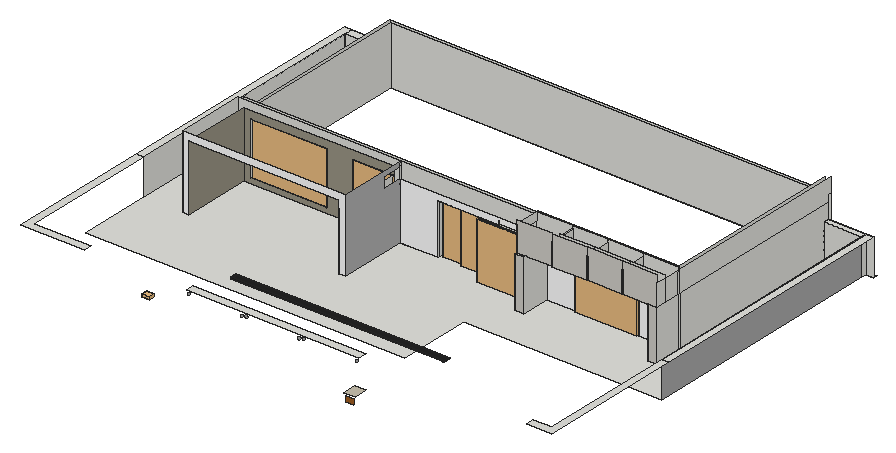
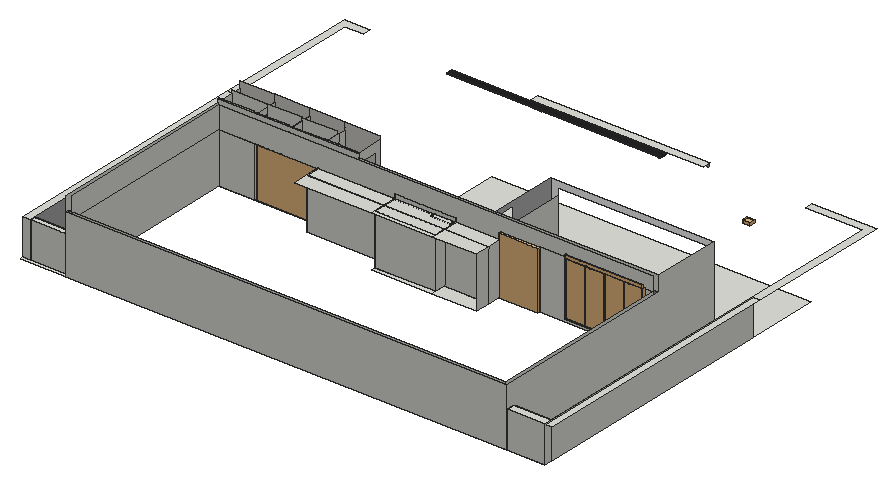
# SketchUp Ruby script. Lengths in inches.
U = 1.inch
M = Sketchup.active_model
def pt(a) = Geom::Point3d.new(a.map { |v| v * U })
def face(e, loops, mat)
  f = e.add_face(loops[0].map { |a| pt(a) })
  loops[1..].each { |l| e.add_face(l.map { |a| pt(a) }).erase! }
  f.material = f.back_material = mat if mat
  f
end
# faces: each face lists its corners as indices into pts; further lists are holes
def faces(e, pts, list, mat = nil) = list.each { |f| face(e, (f[0].is_a?(Array) ? f : [f]).map { |l| l.map { |i| pts[i] } }, mat) }
# xy, xz, yz: faces in a plane at the given z, y or x. An outline is a flat list of corners, or four numbers for a rectangle; further outlines are holes
def ring(l) = l.size == 4 ? [[l[0], l[1]], [l[2], l[1]], [l[2], l[3]], [l[0], l[3]]] : l.each_slice(2).to_a
def flat(e, list, mat, &to3) = list.each { |f| face(e, (f[0].is_a?(Array) ? f : [f]).map { |l| ring(l).map { |u, v| to3.(u, v) } }, mat) }
def xy(e, z, list, mat = nil) = flat(e, list, mat) { |x, y| [x, y, z] }
def xz(e, y, list, mat = nil) = flat(e, list, mat) { |x, z| [x, y, z] }
def yz(e, x, list, mat = nil) = flat(e, list, mat) { |y, z| [x, y, z] }
def lines(e, pts, list) = list.each { |a, b| e.add_line(pt(pts[a]), pt(pts[b])) }
# prism: a flat outline (further loops are holes) pulled along v
def prism(e, loops, v, mat = nil)
  f = face(e, loops, mat); d = Geom::Vector3d.new(v.map { |x| x * U })
  f.pushpull(f.normal.samedirection?(d) ? d.length : -d.length)
end
def box(e, o, s, mat = nil) = prism(e, [[o, [o[0] + s[0], o[1], o[2]], [o[0] + s[0], o[1] + s[1], o[2]], [o[0], o[1] + s[1], o[2]]]], [0, 0, s[2]], mat)
def at(x, y, z, deg = 0) = Geom::Transformation.translation(pt([x, y, z])) * Geom::Transformation.rotation(ORIGIN, Z_AXIS, deg.degrees)
def axes(o, x, y, z) = Geom::Transformation.new([*x, 0, *y, 0, *z, 0, *pt(o).to_a, 1])
def part(name) = M.definitions.add(name)
# library, detail: a bought-in or finely detailed component or shape, given as its bounding box
def library(name, o, s) = part(name).tap { |d| box(d.entities, o, s) }
def detail(e, o, s) = box(e.add_group.entities, o, s)
def put(e, d, t, mat = nil) = e.add_instance(d, t).tap { |i| i.material = mat if mat }
def group(e, t, mat = nil) = e.add_group.tap { |g| g.transformation = t; g.material = mat if mat }.entities
root = M.entities
M.materials.add("Material~3").color = [123, 113, 102]
M.materials.add("[0128_White]").color = [255, 255, 255]
M.materials.add("[0129_WhiteSmoke]").color = [178, 178, 178]
M.materials.add("[0132_LightGray]").color = [169, 169, 169]
M.materials.add("[0136_Charcoal]").color = [35, 35, 35]
M.materials.add("[Concrete Tile]").color = [155, 150, 134]
M.materials.add("[Terrazzo Tile Light]").color = [209, 207, 200]
M.materials.add("[Tile Canvas]").color = [199, 192, 173]
M.materials.add("[Wood Square Tile 02]").color = [160, 95, 34]
M.materials.add("terracota").color = [125, 74, 68]
c1 = library("3DGeom~4_Defintion",[362.52,-15.59,12.6],[288.85,70.11,1000])
c2 = library("3 door",[0,0,0],[74.8,3.9375,43.31])
c3 = library("Shallow planter bowl",[0,0,0],[21.33,16.65,7.48])
c4 = library("door (1)",[38.93,25.48,0],[40,9.94,82.68])
c5 = part("Group\#105")
prism(c5.entities,[[[353.71,0,0.79],[353.71,0,-1.18],[353.71,10.43,-1.18],[353.71,10.43,0.79],[353.71,10.12,0.79],[353.71,10.12,0.39],[353.71,7.09,0.39],[353.71,7.09,0.79],[353.71,6.73,0.79],[353.71,6.73,0.39],[353.71,3.7,0.39],[353.71,3.7,0.79],[353.71,3.35,0.79],[353.71,3.35,0.39],[353.71,0.31,0.39],[353.71,0.31,0.79]]],[-353.71,0,0])
c6 = library("JALI+PATTERN-03",[8.875,53.125,6.4375],[84,1,53.5])
xy(root,5.1875,[[[2928.38,611.53,3456.29,611.53,3456.29,732.28,3784.01,732.28,3784.01,1146.63,3720.76,1146.63,3720.76,851.0625,3551.34,851.0625,3551.34,845.35,3503.88,845.35,3503.88,798.41,3488.55,798.41,3488.55,845.35,3424.27,845.35,3424.27,874.25,3323.99,874.25,3323.99,845.35,3261.3,845.35,3261.3,732.28,3250.36,732.28,3250.36,851.0625,3184.99,851.0625,3184.99,845.35,3002.95,845.35,3002.95,732.28,2992.01,732.28,2992.01,1146.63,2928.38,1146.63],[3705.43,801.78,3720.76,845.35]],[2992.01,732.28,2992.01,1160.85,3796.01,1160.85,3796.01,1155.13,2997.72,1155.13,2997.72,851.0625,3184.99,851.0625,3184.99,845.35,3002.95,845.35,3002.95,732.28],[3250.36,732.28,3250.36,846.1,3323.99,846.1,3323.99,845.35,3261.3,845.35,3261.3,732.28],[3488.55,798.41,3488.55,845.35,3424.27,845.35,3424.27,846.1,3551.34,846.1,3551.34,845.35,3503.88,845.35,3503.88,798.41],[3705.43,801.78,3720.76,845.35],
  [3250.36,846.1,3323.99,874.25],[3424.27,846.1,3551.34,874.25],[3715.04,851.0625,3720.76,1155.13],[3250.36,874.25,3323.99,900.375],[3323.99,874.25,3424.27,892.35],
  [3323.99,892.35,3424.27,900.375],[2928.38,1146.63,2992.01,1160.85],[3720.76,1146.63,3784.01,1155.13]])
xy(root,13.84,[[3014.67,845.35,3139.54,851.0625]])
xy(root,32.74,[[3482.52,453.42,3500.96,475.99]],"[Tile Canvas]")
xy(root,65.1875,[[2916.76,491.47,3022.65,491.47,3022.65,505.1,2928.38,505.1,2928.38,732.28,2916.76,732.28],[3191.65,491.47,3476.5,505.1],[3753.3125,491.47,3796.01,491.47,3796.01,732.28,3784.01,732.28,3784.01,505.1,3753.3125,505.1],[2916.76,732.28,2928.38,1160.85],[3784.01,732.28,3796.01,1155.13],
  [2928.38,1146.63,2992.01,1160.85],[3720.76,1146.63,3784.01,1155.13]])
xy(root,89.42,[[3488.55,798.41,3503.88,801.78],[3503.88,801.78,3546.61,814.22],[3547.54,801.78,3551.34,817.6],[3551.34,801.78,3604.66,817.6],[3605.72,801.78,3655.96,817.6],
  [3655.96,801.78,3662.71,817.6],[3664.02,801.78,3705.43,817.6],[3705.43,801.78,3720.76,817.6],[3503.88,814.22,3546.61,844.47],[3547.54,817.6,3551.34,844.47],
  [3551.34,817.6,3604.66,844.47],[3605.72,817.6,3655.96,844.47],[3655.96,817.6,3662.71,844.47],[3664.02,817.6,3705.43,844.47],[3705.43,817.6,3720.76,844.47],
  [3488.55,844.47,3503.88,845.35],[3503.88,844.47,3551.34,845.35],[3551.34,844.47,3655.96,845.35],[3655.96,844.47,3705.43,845.35],[3705.43,844.47,3720.76,845.35],
  [3323.99,845.35,3424.27,846.1],[3424.27,845.35,3488.55,846.1],[3488.55,845.35,3551.34,846.1],[3551.34,845.35,3655.96,846.1],[3655.96,845.35,3720.76,846.1],
  [3250.36,846.1,3323.99,851.0625],[3424.27,846.1,3551.34,851.0625],[3551.34,846.1,3655.96,851.0625],[3655.96,846.1,3720.76,851.0625],[3250.36,851.0625,3323.99,874.25],
  [3323.99,851.0625,3424.27,874.25],[3424.27,851.0625,3551.34,874.25],[3715.04,851.0625,3720.76,1155.13],[3250.36,874.25,3323.99,900.375],[3323.99,874.25,3424.27,892.35],
  [3424.27,874.25,3551.34,900.375],[3323.99,892.35,3424.27,900.375]])
xz(root,453.42,[[3484.87,19.53,3499,29.34]],"[Wood Square Tile 02]")
xz(root,491.47,[[3282.87,57.74,3283.35,57.8,3283.8,57.99,3284.19,58.29,3284.49,58.68,3284.68,59.13,3284.74,59.61,3284.68,60.1,3284.49,60.55,3284.19,60.94,3283.8,61.24,3283.35,61.43,3282.87,61.49,3282.38,61.43,3281.93,61.24,3281.54,60.94,3281.24,60.55,3281.06,60.1,3280.99,59.61,3281.06,59.13,3281.24,58.68,3281.54,58.29,3281.93,57.99,3282.38,57.8],[3377.82,57.74,3378.3,57.8,3378.76,57.99,3379.14,58.29,3379.44,58.68,3379.63,59.13,3379.69,59.61,3379.63,60.1,3379.44,60.55,3379.14,60.94,3378.76,61.24,3378.3,61.43,3377.82,61.49,3377.33,61.43,3376.88,61.24,3376.49,60.94,3376.19,60.55,3376.01,60.1,3375.94,59.61,3376.01,59.13,3376.19,58.68,3376.49,58.29,3376.88,57.99,3377.33,57.8],[3472.77,57.74,3473.25,57.8,3473.71,57.99,3474.09,58.29,3474.39,58.68,3474.58,59.13,3474.64,59.61,3474.58,60.1,3474.39,60.55,3474.09,60.94,3473.71,61.24,3473.25,61.43,3472.77,61.49,3472.28,61.43,3471.83,61.24,3471.44,60.94,3471.15,60.55,3470.96,60.1,3470.89,59.61,3470.96,59.13,3471.15,58.68,3471.44,58.29,3471.83,57.99,3472.28,57.8],[3195.13,59.21,3195.625,59.22,3196.09,59.36,3196.51,59.61,3196.85,59.97,3197.08,60.4,3197.2,60.875,3197.1875,61.36,3197.05,61.83,3196.79,62.25,3196.4375,62.59,3196.01,62.82,3195.53,62.9375,3195.04,62.93,3194.57,62.79,3194.16,62.53,3193.82,62.18,3193.58,61.75,3193.47,61.27,3193.48,60.78,3193.62,60.32,3193.875,59.9,3194.23,59.56,3194.66,59.33],[3290.09,59.21,3290.57,59.22,3291.04,59.36,3291.46,59.61,3291.8,59.97,3292.03,60.4,3292.15,60.875,3292.14,61.36,3292,61.83,3291.74,62.25,3291.39,62.59,3290.96,62.82,3290.48,62.9375,3290,62.93,3289.53,62.79,3289.11,62.53,3288.77,62.18,3288.54,61.75,3288.42,61.27,3288.43,60.78,3288.57,60.32,3288.83,59.9,3289.18,59.56,3289.61,59.33],
  [3385.04,59.21,3385.53,59.22,3385.99,59.36,3386.41,59.61,3386.75,59.97,3386.98,60.4,3387.1,60.875,3387.09,61.36,3386.95,61.83,3386.7,62.25,3386.34,62.59,3385.91,62.82,3385.44,62.9375,3384.95,62.93,3384.48,62.79,3384.06,62.53,3383.72,62.18,3383.49,61.75,3383.37,61.27,3383.38,60.78,3383.52,60.32,3383.78,59.9,3384.13,59.56,3384.56,59.33]],"[0132_LightGray]")
xz(root,732.28,[[2992.01,5.1875,3002.95,5.1875,3002.95,114.25,3250.36,114.25,3250.36,5.1875,3261.3,5.1875,3261.3,125.1875,2992.01,125.1875]],"[0128_White]")
xz(root,798.41,[[3488.55,5.1875,3503.88,89.42]],"[Terrazzo Tile Light]")
xz(root,801.78,[[3705.43,5.1875,3720.76,89.42],[[3488.55,89.42,3546.61,138.0625],[3492.44,131.88,3492.15,131.92,3491.88,132.03,3491.65,132.21,3491.47,132.44,3491.35,132.71,3491.32,133,3491.35,133.29,3491.47,133.57,3491.65,133.8,3491.88,133.98,3492.15,134.09,3492.44,134.13,3492.73,134.09,3493,133.98,3493.24,133.8,3493.41,133.57,3493.53,133.29,3493.57,133,3493.53,132.71,3493.41,132.44,3493.24,132.21,3493,132.03,3492.73,131.92],[3543.57,131.88,3543.27,131.92,3543,132.03,3542.77,132.21,3542.59,132.44,3542.48,132.71,3542.44,133,3542.48,133.29,3542.59,133.57,3542.77,133.8,3543,133.98,3543.27,134.09,3543.57,134.13,3543.86,134.09,3544.13,133.98,3544.36,133.8,3544.54,133.57,3544.65,133.29,3544.69,133,3544.65,132.71,3544.54,132.44,3544.36,132.21,3544.13,132.03,3543.86,131.92],[3543.57,91.63,3543.27,91.67,3543,91.78,3542.77,91.96,3542.59,92.19,3542.48,92.46,3542.44,92.75,3542.48,93.04,3542.59,93.32,3542.77,93.55,3543,93.73,3543.27,93.84,3543.57,93.88,3543.86,93.84,3544.13,93.73,3544.36,93.55,3544.54,93.32,3544.65,93.04,3544.69,92.75,3544.65,92.46,3544.54,92.19,3544.36,91.96,3544.13,91.78,3543.86,91.67],[3491.38,91.63,3491.09,91.67,3490.82,91.78,3490.58,91.96,3490.4,92.19,3490.29,92.46,3490.25,92.75,3490.29,93.04,3490.4,93.32,3490.58,93.55,3490.82,93.73,3491.09,93.84,3491.38,93.88,3491.67,93.84,3491.94,93.73,3492.17,93.55,3492.35,93.32,3492.46,93.04,3492.5,92.75,3492.46,92.46,3492.35,92.19,3492.17,91.96,3491.94,91.78,3491.67,91.67]],[[3547.54,89.42,3604.66,138.0625],[3551.43,131.88,3551.14,131.92,3550.87,132.03,3550.63,132.21,3550.45,132.44,3550.34,132.71,3550.3,133,3550.34,133.29,3550.45,133.57,3550.63,133.8,3550.87,133.98,3551.14,134.09,3551.43,134.13,3551.72,134.09,3551.99,133.98,3552.22,133.8,3552.4,133.57,3552.52,133.29,3552.55,133,3552.52,132.71,3552.4,132.44,3552.22,132.21,3551.99,132.03,3551.72,131.92],[3602.55,91.63,3602.26,91.67,3601.99,91.78,3601.76,91.96,3601.58,92.19,3601.47,92.46,3601.43,92.75,3601.47,93.04,3601.58,93.32,3601.76,93.55,3601.99,93.73,3602.26,93.84,3602.55,93.88,3602.85,93.84,3603.12,93.73,3603.35,93.55,3603.53,93.32,3603.64,93.04,3603.68,92.75,3603.64,92.46,3603.53,92.19,3603.35,91.96,3603.12,91.78,3602.85,91.67],[3550.37,91.63,3550.08,91.67,3549.8,91.78,3549.57,91.96,3549.39,92.19,3549.28,92.46,3549.24,92.75,3549.28,93.04,3549.39,93.32,3549.57,93.55,3549.8,93.73,3550.08,93.84,3550.37,93.88,3550.66,93.84,3550.93,93.73,3551.16,93.55,3551.34,93.32,3551.45,93.04,3551.49,92.75,3551.45,92.46,3551.34,92.19,3551.16,91.96,3550.93,91.78,3550.66,91.67],[3602.55,131.88,3602.26,131.92,3601.99,132.03,3601.76,132.21,3601.58,132.44,3601.47,132.71,3601.43,133,3601.47,133.29,3601.58,133.57,3601.76,133.8,3601.99,133.98,3602.26,134.09,3602.55,134.13,3602.85,134.09,3603.12,133.98,3603.35,133.8,3603.53,133.57,3603.64,133.29,3603.68,133,3603.64,132.71,3603.53,132.44,3603.35,132.21,3603.12,132.03,3602.85,131.92]],[[3605.72,89.42,3662.71,138.0625],[3660.73,131.88,3660.4375,131.92,3660.17,132.03,3659.93,132.21,3659.76,132.44,3659.64,132.71,3659.6,133,3659.64,133.29,3659.76,133.57,3659.93,133.8,3660.17,133.98,3660.4375,134.09,3660.73,134.13,3661.02,134.09,3661.29,133.98,3661.53,133.8,3661.7,133.57,3661.82,133.29,3661.85,133,3661.82,132.71,3661.7,132.44,3661.53,132.21,3661.29,132.03,3661.02,131.92],[3609.6,131.88,3609.3125,131.92,3609.04,132.03,3608.81,132.21,3608.63,132.44,3608.52,132.71,3608.48,133,3608.52,133.29,3608.63,133.57,3608.81,133.8,3609.04,133.98,3609.3125,134.09,3609.6,134.13,3609.9,134.09,3610.17,133.98,3610.4,133.8,3610.58,133.57,3610.69,133.29,3610.73,133,3610.69,132.71,3610.58,132.44,3610.4,132.21,3610.17,132.03,3609.9,131.92],[3660.73,91.63,3660.4375,91.67,3660.17,91.78,3659.93,91.96,3659.76,92.19,3659.64,92.46,3659.6,92.75,3659.64,93.04,3659.76,93.32,3659.93,93.55,3660.17,93.73,3660.4375,93.84,3660.73,93.88,3661.02,93.84,3661.29,93.73,3661.53,93.55,3661.7,93.32,3661.82,93.04,3661.85,92.75,3661.82,92.46,3661.7,92.19,3661.53,91.96,3661.29,91.78,3661.02,91.67],[3608.54,91.63,3608.25,91.67,3607.98,91.78,3607.75,91.96,3607.57,92.19,3607.46,92.46,3607.42,92.75,3607.46,93.04,3607.57,93.32,3607.75,93.55,3607.98,93.73,3608.25,93.84,3608.54,93.88,3608.83,93.84,3609.1,93.73,3609.34,93.55,3609.52,93.32,3609.63,93.04,3609.67,92.75,3609.63,92.46,3609.52,92.19,3609.34,91.96,3609.1,91.78,3608.83,91.67]],[[3664.02,89.42,3720.76,138.0625],[3666.84,91.63,3666.55,91.67,3666.28,91.78,3666.05,91.96,3665.87,92.19,3665.76,92.46,3665.72,92.75,3665.76,93.04,3665.87,93.32,3666.05,93.55,3666.28,93.73,3666.55,93.84,3666.84,93.88,3667.13,93.84,3667.41,93.73,3667.64,93.55,3667.82,93.32,3667.93,93.04,3667.97,92.75,3667.93,92.46,3667.82,92.19,3667.64,91.96,3667.41,91.78,3667.13,91.67],[3667.91,131.88,3667.61,131.92,3667.34,132.03,3667.11,132.21,3666.93,132.44,3666.82,132.71,3666.78,133,3666.82,133.29,3666.93,133.57,3667.11,133.8,3667.34,133.98,3667.61,134.09,3667.91,134.13,3668.2,134.09,3668.47,133.98,3668.7,133.8,3668.88,133.57,3668.99,133.29,3669.03,133,3668.99,132.71,3668.88,132.44,3668.7,132.21,3668.47,132.03,3668.2,131.92],[3719.03,91.63,3718.74,91.67,3718.47,91.78,3718.24,91.96,3718.06,92.19,3717.94,92.46,3717.91,92.75,3717.94,93.04,3718.06,93.32,3718.24,93.55,3718.47,93.73,3718.74,93.84,3719.03,93.88,3719.32,93.84,3719.59,93.73,3719.83,93.55,3720,93.32,3720.12,93.04,3720.16,92.75,3720.12,92.46,3720,92.19,3719.83,91.96,3719.59,91.78,3719.32,91.67],[3719.03,131.88,3718.74,131.92,3718.47,132.03,3718.24,132.21,3718.06,132.44,3717.94,132.71,3717.91,133,3717.94,133.29,3718.06,133.57,3718.24,133.8,3718.47,133.98,3718.74,134.09,3719.03,134.13,3719.32,134.09,3719.59,133.98,3719.83,133.8,3720,133.57,3720.12,133.29,3720.16,133,3720.12,132.71,3720,132.44,3719.83,132.21,3719.59,132.03,3719.32,131.92]]],"[Terrazzo Tile Light]")
xz(root,817.6,[[3547.54,89.42,3604.66,131.1875],[3605.72,89.42,3662.71,131.1875],[3664.02,89.42,3720.76,131.1875]])
xz(root,844.47,[[3488.55,89.42,3546.61,131.1875],[3546.61,89.42,3547.54,131.1875],[3547.54,89.42,3604.66,131.1875],[3604.66,89.42,3605.72,131.1875],[3605.72,89.42,3662.71,131.1875],
  [3662.71,89.42,3664.02,131.1875],[3664.02,89.42,3720.76,131.1875]])
xz(root,845.35,[[3424.27,5.1875,3488.55,89.42],[3705.43,5.1875,3720.76,89.42]])
xz(root,845.35,[[3261.3,5.1875,3323.99,5.1875,3323.99,89.42,3488.55,89.42,3488.55,99.26,3261.3,99.26],[3503.88,5.1875,3551.34,89.42],[3655.96,5.1875,3705.43,89.42]],"[0128_White]")
xz(root,845.35,[[[3002.95,5.1875,3184.99,5.1875,3184.99,101.375,3250.36,101.375,3250.36,114.25,3002.95,114.25],[3014.67,13.84,3139.54,101.78]]],"[Concrete Tile]")
xz(root,846.1,[[3250.36,5.1875,3323.99,89.42],[3424.27,5.1875,3551.34,89.42],[3250.36,89.42,3261.3,89.42,3261.3,125.1875,2992.01,125.1875,2992.01,101.375,3250.36,101.375],[3261.3,89.42,3261.3,125.1875,3488.55,125.1875,3488.55,89.42,3424.27,89.42,3424.27,95.79,3323.99,95.79,3323.99,89.42],[3323.99,89.42,3424.27,95.79],
  [3488.55,89.42,3720.76,131.1875]])
xz(root,851.0625,[[2997.72,5.1875,2997.72,101.375,3014.67,101.375,3014.67,13.84,3139.54,13.84,3139.54,101.375,3184.99,101.375,3184.99,5.1875],[3655.96,5.1875,3715.04,89.42],[3715.04,5.1875,3720.76,89.42],[3250.36,89.42,3250.36,101.375,3139.54,101.375,3139.54,101.78,3014.67,101.78,3014.67,101.375,2997.72,101.375,2997.72,125.1875,3715.04,125.1875,3715.04,89.42,3424.27,89.42,3424.27,95.79,3323.99,95.79,3323.99,89.42],[3323.99,89.42,3424.27,95.79]])
xz(root,874.25,[[3250.36,5.1875,3551.34,89.42]])
xz(root,892.35,[[3323.99,5.1875,3424.27,89.42]])
xz(root,1146.63,[[2928.38,5.1875,2992.01,65.1875],[3720.76,5.1875,3784.01,65.1875]])
xz(root,1155.13,[[2997.72,5.1875,3715.04,101.375],[3715.04,5.1875,3720.76,89.42],[3720.76,5.1875,3784.01,65.1875],[3784.01,5.1875,3796.01,65.1875],[3715.04,89.42,3720.76,101.375]])
xz(root,1160.85,[[2928.38,5.1875,2992.01,65.1875],[2992.01,5.1875,3720.76,101.375]])
yz(root,2928.38,[[732.28,5.1875,1146.63,65.1875],[1146.63,5.1875,1160.85,65.1875]])
yz(root,2992.01,[[732.28,5.1875,732.28,125.1875,846.1,125.1875,846.1,101.375,1160.85,101.375,1160.85,65.1875,1146.63,65.1875,1146.63,5.1875],[1146.63,5.1875,1160.85,65.1875]])
yz(root,2997.72,[[851.0625,5.1875,1155.13,101.375]])
yz(root,3002.95,[[732.28,5.1875,845.35,114.25]],"[Concrete Tile]")
yz(root,3014.67,[[845.35,13.84,851.0625,101.78]])
yz(root,3139.54,[[845.35,13.84,851.0625,101.78]])
yz(root,3184.99,[[845.35,5.1875,851.0625,101.375]])
yz(root,3250.36,[[732.28,5.1875,846.1,101.375],[846.1,5.1875,874.25,89.42],[874.25,5.1875,900.375,89.42],[846.1,89.42,851.0625,101.375]])
yz(root,3261.3,[[845.35,89.42,846.1,125.1875]])
yz(root,3261.3,[[732.28,5.1875,845.35,5.1875,845.35,99.26,810.97,99.26,810.97,117.26,845.35,117.26,845.35,125.1875,732.28,125.1875]],"[0129_WhiteSmoke]")
yz(root,3323.99,[[845.35,5.1875,846.1,89.42],[846.1,5.1875,892.35,89.42],[846.1,89.42,851.0625,95.79]])
yz(root,3424.27,[[845.35,5.1875,846.1,89.42],[846.1,5.1875,892.35,89.42],[846.1,89.42,851.0625,95.79]])
yz(root,3488.55,[[798.41,5.1875,798.41,89.42,801.78,89.42,801.78,131.1875,844.47,131.1875,844.47,117.26,810.97,117.26,810.97,99.26,844.47,99.26,844.47,89.42,845.35,89.42,845.35,5.1875],[844.47,89.42,845.35,99.26],[845.35,89.42,846.1,125.1875]])
yz(root,3503.88,[[798.41,5.1875,845.35,89.42]])
yz(root,3546.61,[[801.78,89.42,814.22,125.1875],[814.22,89.42,844.47,125.1875]])
yz(root,3547.54,[[801.78,89.42,817.6,125.1875],[817.6,89.42,844.47,125.1875]])
yz(root,3551.34,[[845.35,5.1875,846.1,89.42],[846.1,5.1875,874.25,89.42]])
yz(root,3604.66,[[801.78,89.42,817.6,125.1875],[817.6,89.42,844.47,125.1875]])
yz(root,3605.72,[[801.78,89.42,817.6,125.1875],[817.6,89.42,844.47,125.1875]])
yz(root,3655.96,[[845.35,5.1875,851.0625,89.42]])
yz(root,3662.71,[[801.78,89.42,817.6,125.1875],[817.6,89.42,844.47,125.1875]])
yz(root,3664.02,[[801.78,89.42,817.6,125.1875],[817.6,89.42,844.47,125.1875]])
yz(root,3705.43,[[801.78,5.1875,845.35,89.42]])
yz(root,3715.04,[[851.0625,5.1875,1155.13,89.42],[851.0625,89.42,1155.13,125.1875]])
yz(root,3720.76,[[801.78,5.1875,845.35,89.42],[851.0625,5.1875,1146.63,5.1875,1146.63,65.1875,1155.13,65.1875,1155.13,89.42,851.0625,89.42],[1146.63,5.1875,1155.13,65.1875],[801.78,89.42,817.6,125.1875],[817.6,89.42,844.47,125.1875],
  [844.47,89.42,846.1,125.1875],[846.1,89.42,1155.13,89.42,1155.13,101.375,1160.85,101.375,1160.85,125.1875,846.1,125.1875]])
yz(root,3784.01,[[1146.63,5.1875,1155.13,65.1875]])
yz(root,3784.01,[[732.28,5.1875,1146.63,65.1875]],"[0132_LightGray]")
p = [[3488.55,814.22,89.42],[3503.88,814.22,89.42]]
lines(root,p,[[0,1]])
put(root,c1,axes([2972.06,853.3125,12.94],[0.11056,0,0],[0,-0.05859,0],[0,0,0.08734]),"Material~3")
put(root,c1,axes([3003.53,853.99,12.94],[0.11056,0,0],[0,-0.05859,0],[0,0,0.08734]),"Material~3")
put(root,c2,axes([3014.67,847.72,10.15],[1.71563,0,0],[0,1.38,0],[0,0,2.21476]))
put(root,c1,axes([3035.6,853.99,12.94],[0.11056,0,0],[0,-0.05859,0],[0,0,0.08734]),"Material~3")
put(root,c3,axes([3114.98,510.84,16.37],[-0.59053,0,0],[0,0.56886,0],[0,0,0.56886]),"terracota")
put(root,c1,axes([3067.66,853.99,12.94],[0.11056,0,0],[0,-0.05859,0],[0,0,0.08734]),"Material~3")
put(root,c4,axes([3121.37,814.19,5.1875],[1.63437,0,0],[0,1.16,0],[0,0,1.16]))
put(root,c1,axes([3286.95,857.09,3.96],[0.11056,0,0],[0,-0.11056,0],[0,0,0.08439]),"Material~3")
put(root,c1,axes([3320.32,851.7,3.96],[0.11056,0,0],[0,-0.08955,0],[0,0,0.08439]),"Material~3")
put(root,c1,axes([3352.26,851.7,3.96],[0.11056,0,0],[0,-0.08955,0],[0,0,0.08439]),"Material~3")
put(root,c5,axes([3232.98,541.01,81.03],[1,0,0],[0,-1,0],[0,0,-1]),"[0136_Charcoal]")
put(root,c6,axes([3393.9,766.91,109.2],[0,0,-1.12],[0,1.12,0],[1.5792,0,0]))
put(root,c2,axes([3551.34,843.85,5.1875],[1.38,0,0],[0,1.38,0],[0,0,1.94496]))
